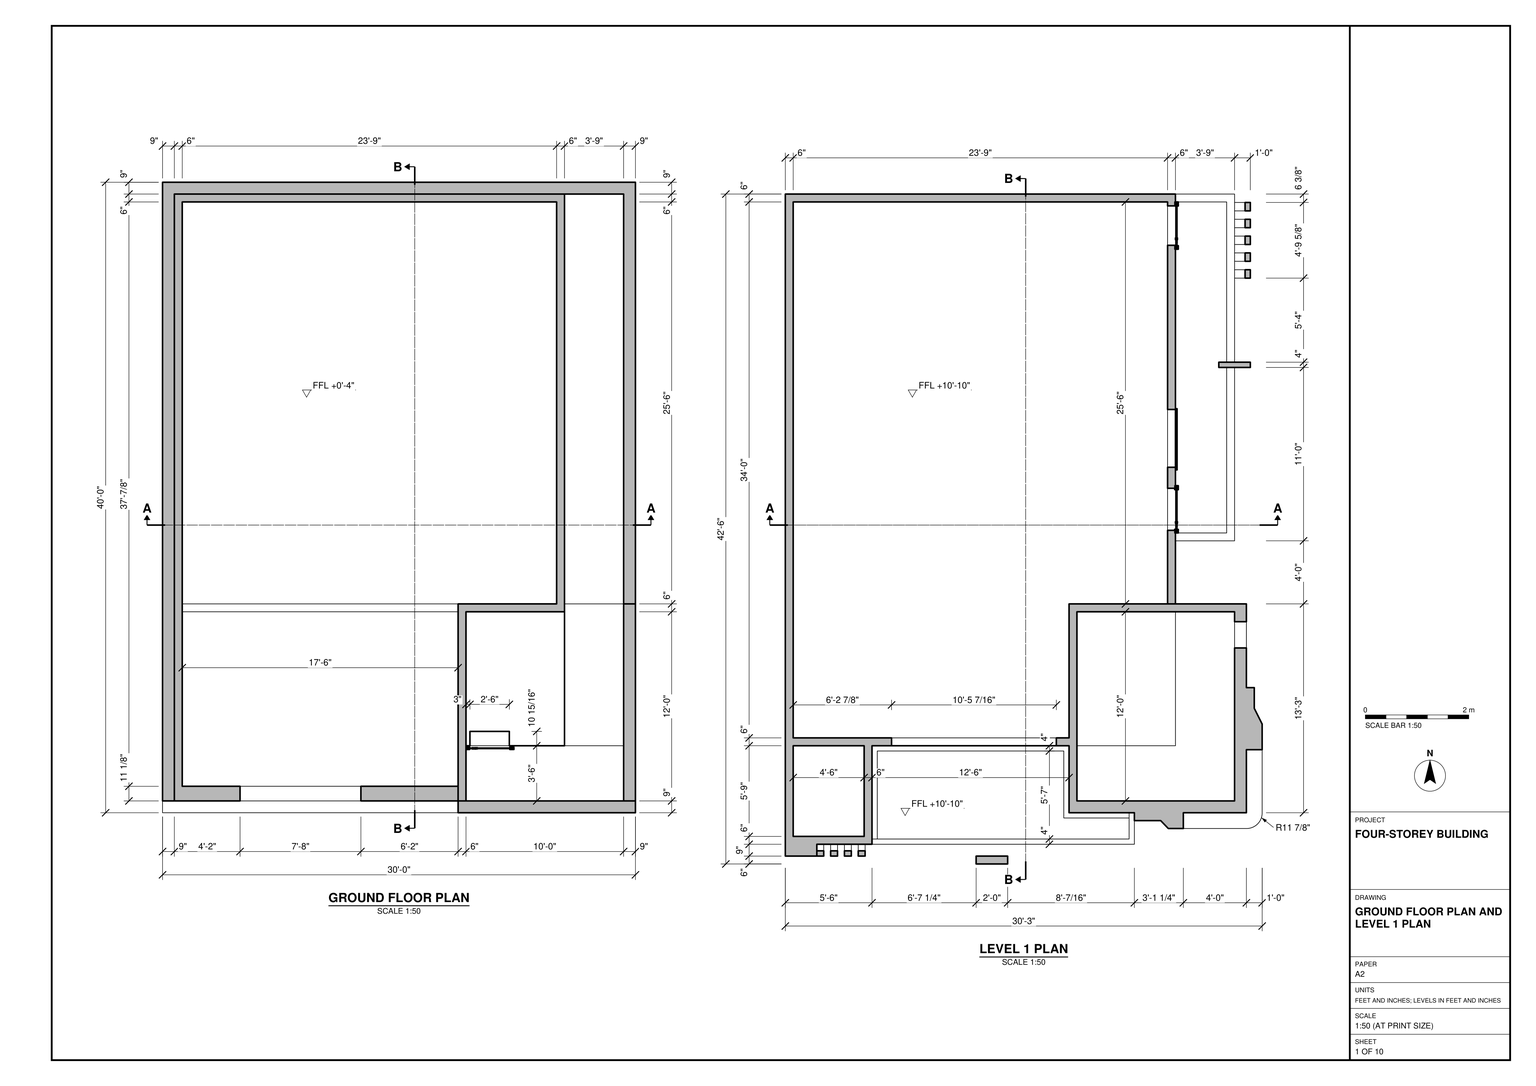
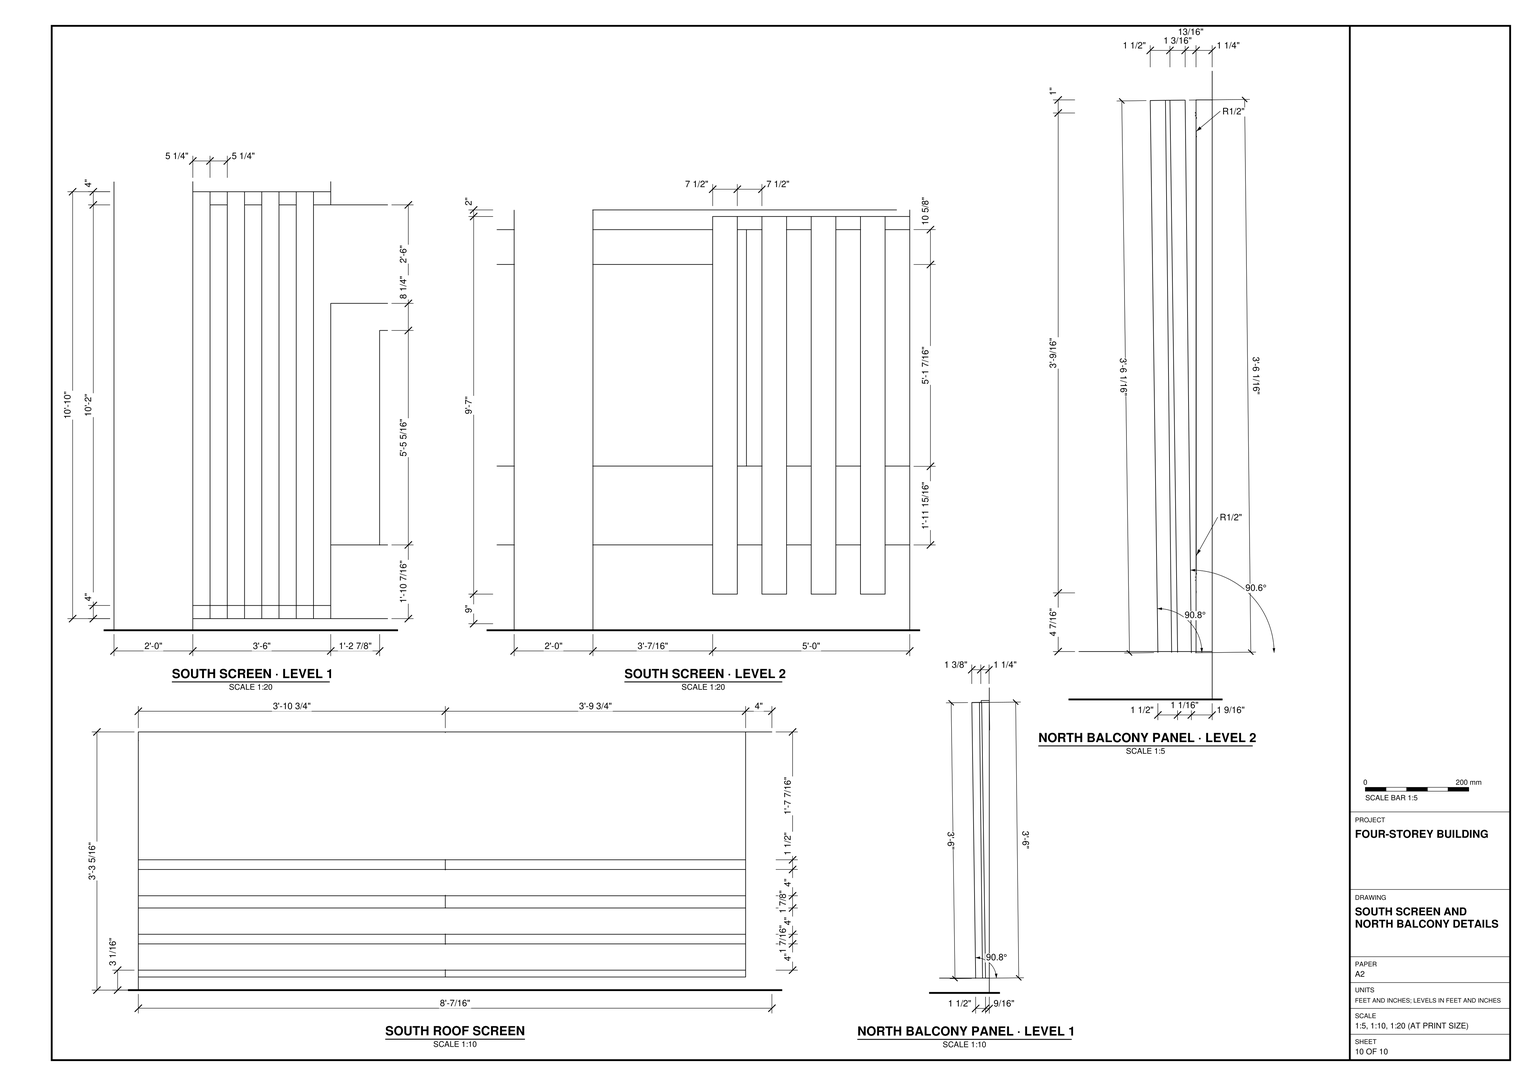
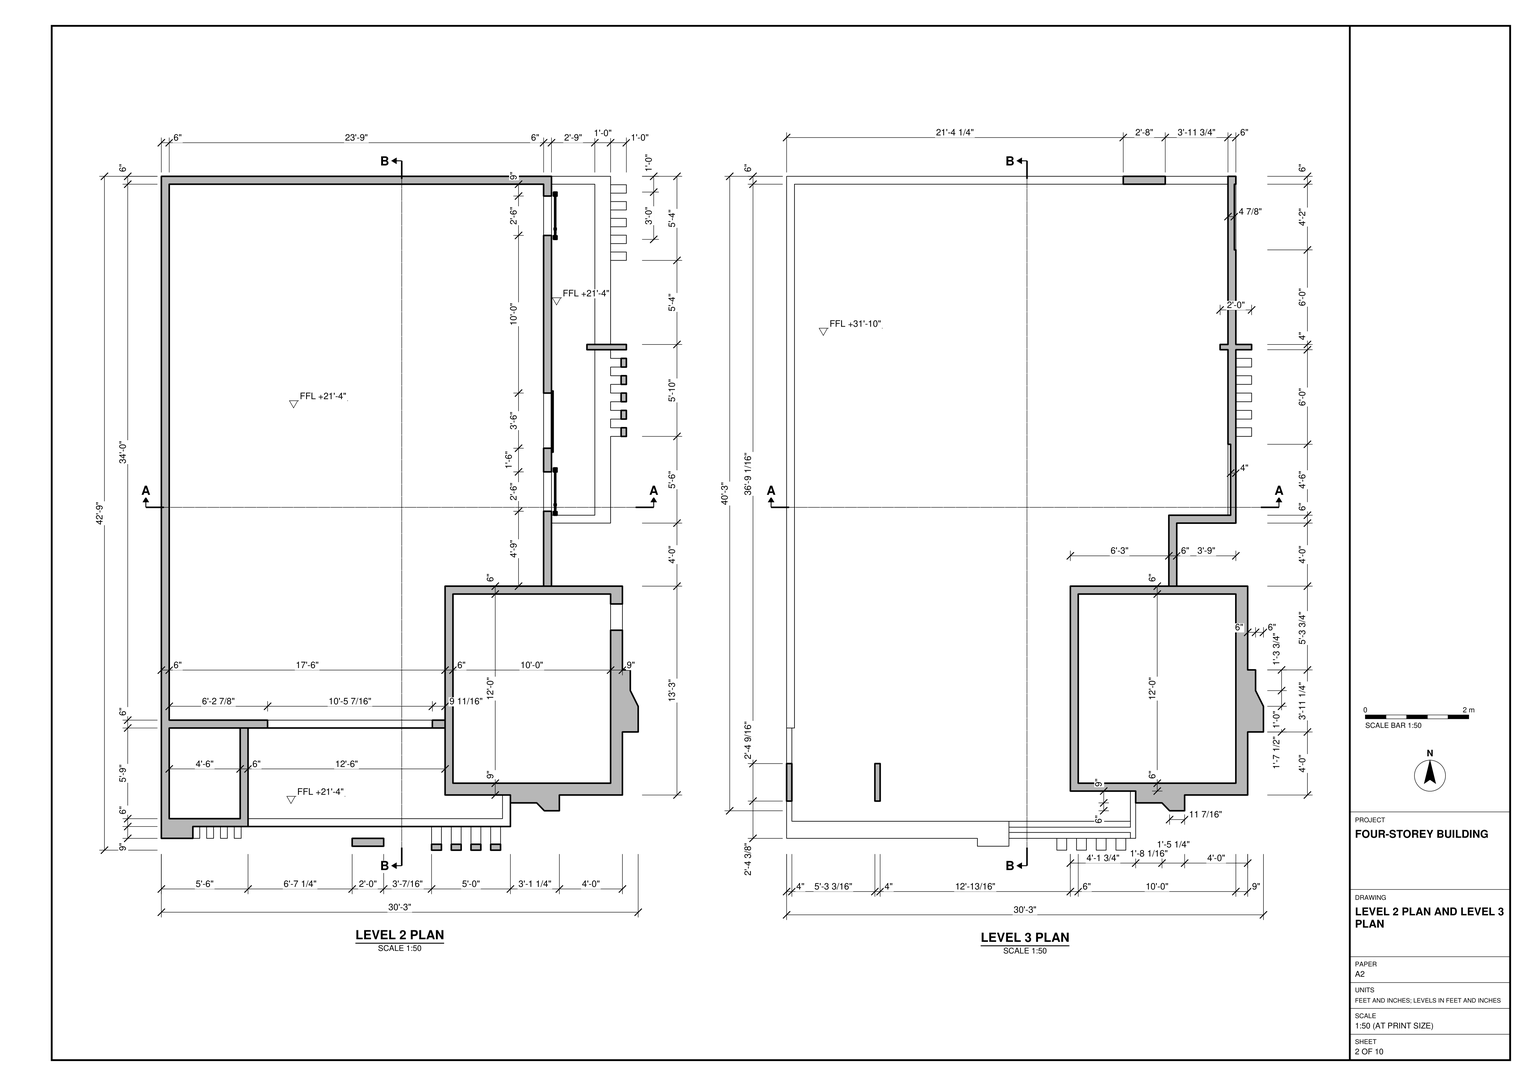
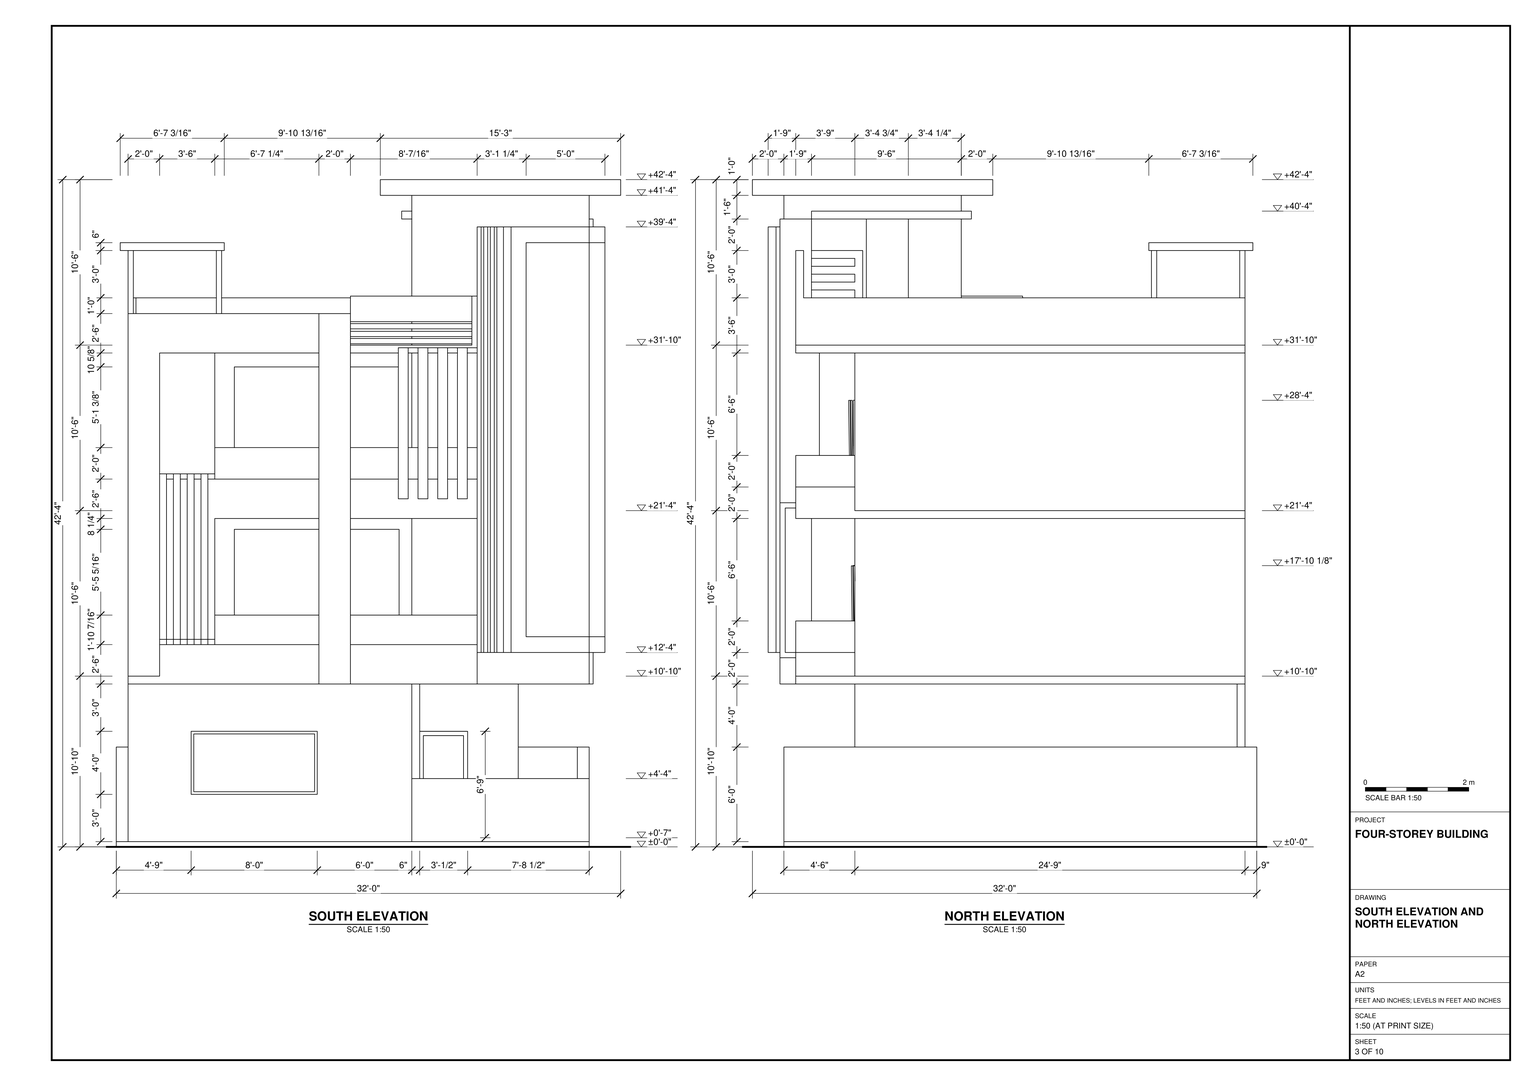
Use task_files/diagram_01.pdf to build the four-storey building in SketchUp. Work in feet and inches. The overall extents, including projections, are 32'-0" east to west, 43'-6" north to south and 42'-4" high. Set the ground datum at ±0'-0" and the upper levels at +10'-10", +21'-4" and +31'-10".

Build each floor from its own plan. Place the wide opening in the south ground-floor wall, align the southeast bay through the upper levels and follow the stepped outline at level 3. Use the wall thicknesses dimensioned on the plans, including 6" and 9" where shown. Place the doors and window units in their drawn openings. Use the plans and sections together for floor slabs, balconies, stairs where shown, and the roof. Match the south screens, south roof screen and north balcony panels to the details on sheet 10; the screen layout changes between levels 1 and 2.

Include built-in joinery and main furniture only where shown. Decor and loose items may be any suitable library components. Keep shell elements such as walls, slabs and roof, and each furniture or joinery piece, in separate groups or components. Use components for repeated parts. Save one SketchUp model as output_files/four_storey_building_with_balconies_and_facade_screens.skp.

# SketchUp Ruby script. Lengths in inches.
U = 1.inch
M = Sketchup.active_model
def pt(a) = Geom::Point3d.new(a.map { |v| v * U })
def face(e, loops, mat)
  f = e.add_face(loops[0].map { |a| pt(a) })
  loops[1..].each { |l| e.add_face(l.map { |a| pt(a) }).erase! }
  f.material = f.back_material = mat if mat
  f
end
# faces: each face lists its corners as indices into pts; further lists are holes
def faces(e, pts, list, mat = nil) = list.each { |f| face(e, (f[0].is_a?(Array) ? f : [f]).map { |l| l.map { |i| pts[i] } }, mat) }
# xy, xz, yz: faces in a plane at the given z, y or x. An outline is a flat list of corners, or four numbers for a rectangle; further outlines are holes
def ring(l) = l.size == 4 ? [[l[0], l[1]], [l[2], l[1]], [l[2], l[3]], [l[0], l[3]]] : l.each_slice(2).to_a
def flat(e, list, mat, &to3) = list.each { |f| face(e, (f[0].is_a?(Array) ? f : [f]).map { |l| ring(l).map { |u, v| to3.(u, v) } }, mat) }
def xy(e, z, list, mat = nil) = flat(e, list, mat) { |x, y| [x, y, z] }
def xz(e, y, list, mat = nil) = flat(e, list, mat) { |x, z| [x, y, z] }
def yz(e, x, list, mat = nil) = flat(e, list, mat) { |y, z| [x, y, z] }
def lines(e, pts, list) = list.each { |a, b| e.add_line(pt(pts[a]), pt(pts[b])) }
# prism: a flat outline (further loops are holes) pulled along v
def prism(e, loops, v, mat = nil)
  f = face(e, loops, mat); d = Geom::Vector3d.new(v.map { |x| x * U })
  f.pushpull(f.normal.samedirection?(d) ? d.length : -d.length)
end
def box(e, o, s, mat = nil) = prism(e, [[o, [o[0] + s[0], o[1], o[2]], [o[0] + s[0], o[1] + s[1], o[2]], [o[0], o[1] + s[1], o[2]]]], [0, 0, s[2]], mat)
def at(x, y, z, deg = 0) = Geom::Transformation.translation(pt([x, y, z])) * Geom::Transformation.rotation(ORIGIN, Z_AXIS, deg.degrees)
def axes(o, x, y, z) = Geom::Transformation.new([*x, 0, *y, 0, *z, 0, *pt(o).to_a, 1])
def part(name) = M.definitions.add(name)
# library, detail: a bought-in or finely detailed component or shape, given as its bounding box
def library(name, o, s) = part(name).tap { |d| box(d.entities, o, s) }
def detail(e, o, s) = box(e.add_group.entities, o, s)
def put(e, d, t, mat = nil) = e.add_instance(d, t).tap { |i| i.material = mat if mat }
def group(e, t, mat = nil) = e.add_group.tap { |g| g.transformation = t; g.material = mat if mat }.entities
root = M.entities
M.materials.add("C03_Honey_Glow").color = [255, 178, 101]
M.materials.add("C05_Golden_Blaze").color = [255, 123, 0]
M.materials.add("Carpet_04_1K").color = [43, 65, 85]
M.materials.add("D01_Frost_White").color = [255, 242, 206]
M.materials.add("Glass_Basic_01").color = [255, 228, 98]
M.materials["Glass_Basic_01"].alpha = 0.25
M.materials.add("M04_Stone_Frost").color = [142, 142, 142]
M.materials.add("Marble_01_1K").color = [230, 221, 211]
M.materials.add("Plywood_08_1K").color = [202, 166, 113]
M.materials.add("ThomThom - Waistcoat1").color = [242, 242, 242]
M.materials.add("ThomThom - Waistcoat2").color = [178, 178, 177]
M.materials.add("Wood_Veneer_15_1K").color = [103, 69, 45]
M.materials.add("mat_03").color = [63, 24, 24]
c1 = library("porta+4",[0.2,-5.42,1.33],[46.55,4.72,83.21])
c2 = library("mesh-164",[-1582.71,-3144.16,-23.22],[2366.42,2227.34,65.81])
c3 = part("Group13")
put(c3.entities,c2,at(294.66,859.51,3.5))
box(root,[201,21,492],[183,204,12],"M04_Stone_Frost")
xy(root,-4,[[0,42,360,522]])
xy(root,414,[[265.28,507,297.25,513]])
xy(root,474,[[217.28,357,339,507],[217.28,507,265.28,513],[265.28,507,297.25,513],[297.25,507,339,519],[217.28,513,297.25,519]])
xy(root,480,[[217.28,357,339,519]],"M04_Stone_Frost")
xz(root,42,[[0,-4,360,0]])
xz(root,357,[[217.28,474,339,480]],"M04_Stone_Frost")
xz(root,507,[[265.28,414,297.25,474]],"mat_03")
xz(root,513,[[265.28,414,297.25,474]],"mat_03")
xz(root,519,[[217.28,474,339,480]],"M04_Stone_Frost")
xz(root,522,[[0,-4,360,0]])
yz(root,0,[[42,-4,522,0]])
yz(root,217.28,[[357,474,519,480]],"M04_Stone_Frost")
yz(root,265.28,[[507,414,513,474]],"mat_03")
yz(root,297.25,[[507,414,513,474]],"mat_03")
yz(root,339,[[357,474,519,480]],"M04_Stone_Frost")
yz(root,360,[[42,-4,522,0]])
g1 = group(root,at(0,42,0),"D01_Frost_White")
box(g1,[15,-18,126],[54,69,120])
xy(g1,0,[[0,0,225,9],[9,9,225,9,225,20.15,15,20.15,15,465,300,465,300,159,225,159,225,51,231,51,231,153,306,153,306,471,9,471],[225,9,231,51],[231,9,351,51],[351,9,360,159],
  [15,20.15,225,153],[231,51,306,153],[306,51,351,159],[15,153,225,159],[15,159,300,465],
  [306,159,351,471]])
xy(g1,3,[[234,51,264,61.91]])
xy(g1,38,[[59,9,151,20.15]])
xy(g1,48,[[225,0,360,9]])
xy(g1,48,[[351,9,360,159]],"Plywood_08_1K")
xy(g1,72,[[0,9,9,9,9,471,351,471,351,159,360,159,360,480,0,480]])
xy(g1,81,[[234,51,264,61.91]])
xy(g1,82,[[59,9,151,20.15]])
xy(g1,120,[[9,-24,9,9,351,9,351,153,306,153,306,159,360,159,360,0,274.72,0,274.72,-24],[9,9,225,9,225,20.15,15,20.15,15,57,9,57],[225,9,231,51],[231,9,231,51,306,51,306,153,351,153,351,9],[15,20.15,15,465,300,465,300,159,225,159,225,20.15],
  [9,57,15,159],[9,159,15,471],[300,159,306,465],[306,207,306,465,351,465,351,343,363,343,363,339,351,339,351,207],[15,465,306,471],
  [306,465,351,471]])
xy(g1,120,[[154.26,-39,178.26,-33]],"M04_Stone_Frost")
xy(g1,126,[[9,-33,33,-24],[75,-20,79,-20,79,47,221,47,221,-4,270.72,-4,270.72,0,225,0,225,51,75,51],[79,-20,270.72,-20,270.72,-4,221,-4,221,47,79,47],[15,57,225,57,225,159,300,159,300,465,15,465],[306,213,345,213,345,339,339,339,339,343,345,343,345,465,306,465]])
xy(g1,128,[[300,215,306,247]])
xy(g1,129,[[300,432,306,462]])
xy(g1,136.09,[[89.88,51,215.3125,57]])
xy(g1,140,[[351,407,363,413.4],[351,419.8,363,426.2],[351,432.6,363,439],[351,445.4,363,451.8],[351,458.2,363,464.6]],"Marble_01_1K")
xy(g1,144,[[300.55,-12,300.55,-6,274.72,-6,274.72,0,360,0,360,95.25,366,95.25,366,79.5,372,67.5,372,-0.38,371.98,-0.76,371.96,-1.13,371.92,-1.51,371.87,-1.88,371.81,-2.26,371.65,-3,371.55,-3.36,371.44,-3.72,371.32,-4.08,371.19,-4.4375,371.05,-4.79,370.9,-5.13,370.73,-5.47,370.55,-5.81,370.37,-6.14,369.97,-6.78,369.75,-7.09,369.52,-7.39,369.29,-7.68,369.04,-7.97,368.79,-8.25,368.25,-8.79,367.97,-9.04,367.68,-9.29,367.39,-9.52,367.09,-9.75,366.78,-9.97,366.14,-10.37,365.81,-10.55,365.47,-10.73,365.13,-10.9,364.79,-11.05,364.4375,-11.19,364.08,-11.32,363.72,-11.44,363.36,-11.55,363,-11.65,362.26,-11.81,361.88,-11.87,361.51,-11.92,361.13,-11.96,360.76,-11.98,360.38,-12],[300.55,-12,294.76,-6,300.55,-6],[306,207,351,207,351,339,345,339,345,213,306,213],[345,343,351,343,351,471,306,471,306,465,345,465],[351,407,359,413.4],
  [351,419.8,359,426.2],[351,432.6,359,439],[351,445.4,359,451.8],[351,458.2,359,464.6]])
xy(g1,150,[[33,-33,38.25,-24],[43.5,-33,48.75,-24],[54,-33,59.25,-24],[64.5,-33,69.75,-24],[75,-24,274.72,-24,274.72,0,270.72,0,270.72,-20,75,-20]])
xy(g1,154,[[33,-29,38.25,-24],[43.5,-29,48.75,-24],[54,-29,59.25,-24],[64.5,-29,69.75,-24]])
xy(g1,156,[[312,-12,360.38,-12,360.76,-11.98,361.13,-11.96,361.51,-11.92,361.88,-11.87,362.26,-11.81,363,-11.65,363.36,-11.55,363.72,-11.44,364.08,-11.32,364.4375,-11.19,364.79,-11.05,365.13,-10.9,365.47,-10.73,365.81,-10.55,366.14,-10.37,366.78,-9.97,367.09,-9.75,367.39,-9.52,367.68,-9.29,367.97,-9.04,368.25,-8.79,368.79,-8.25,369.04,-7.97,369.29,-7.68,369.52,-7.39,369.75,-7.09,369.97,-6.78,370.37,-6.14,370.55,-5.81,370.73,-5.47,370.9,-5.13,371.05,-4.79,371.19,-4.4375,371.32,-4.08,371.44,-3.72,371.55,-3.36,371.65,-3,371.81,-2.26,371.87,-1.88,371.92,-1.51,371.96,-1.13,371.98,-0.76,372,-0.38,372,48,360,48,360,0,312,0]],"M04_Stone_Frost")
xy(g1,158,[[351,125.45,360,145.45]])
xy(g1,164,[[300,263,306,307]])
xy(g1,202,[[351,125.45,360,145.45]])
xy(g1,207,[[300,432,306,462]])
xy(g1,208,[[300,215,306,247],[300,263,306,307]])
xy(g1,237.75,[[89.88,51,215.3125,57]])
xy(g1,246,[[9,57,15,159],[15,57,15,465,300,465,300,159,225,159,225,57],[9,159,15,471],[300,159,306,465],[15,465,306,471],
  [306,465,351,471]])
xy(g1,246,[[75,-24,75,51,225,51,225,0,274.72,0,274.72,-24]],"C05_Golden_Blaze")
xy(g1,246,[[306,207,306,465,351,465,351,343,339,343,339,339,351,339,351,207]],"Wood_Veneer_15_1K")
xy(g1,252,[[15,-18,69,51],[75,-18,268.72,-18,268.72,0,225,0,225,51,75,51],[15,57,225,57,225,159,300,159,300,465,15,465],[306,213,339,213,339,339,333,339,333,343,339,343,339,465,306,465]])
xy(g1,254,[[351,407,359,413.4],[351,419.8,359,426.2],[351,432.6,359,439],[351,445.4,359,451.8],[351,458.2,359,464.6]])
xy(g1,255,[[300,216,306,246],[300,426,306,456]])
xy(g1,258,[[351,407,363,413.4],[351,419.8,363,426.2],[351,432.6,363,439],[351,445.4,363,451.8],[351,458.2,363,464.6]])
xy(g1,259.73,[[89.88,51,215.3125,57]])
xy(g1,261,[[214.71,-42,222.21,-24],[229.72,-42,237.22,-24],[244.72,-42,252.22,-24],[259.72,-42,267.22,-24]])
xy(g1,265,[[214.71,-37.5,222.21,-24],[229.72,-37.5,237.22,-24],[244.72,-37.5,252.22,-24],[259.72,-37.5,267.22,-24]])
xy(g1,266,[[351,273,363,279.6],[351,286.2,363,292.8],[351,299.4,363,306],[351,312.6,363,319.2],[351,325.8,363,332.4]])
xy(g1,270,[[339,343,351,343,351,471,306,471,306,465,339,465]])
xy(g1,270,[[306,207,351,207,351,273,359,273,359,279.6,351,279.6,351,286.2,359,286.2,359,292.8,351,292.8,351,299.4,359,299.4,359,306,351,306,351,312.6,359,312.6,359,319.2,351,319.2,351,325.8,359,325.8,359,332.4,351,332.4,351,339,339,339,339,213,306,213]],"D01_Frost_White")
xy(g1,276,[[33,-29,38.25,-24],[43.5,-29,48.75,-24],[54,-29,59.25,-24],[64.5,-29,69.75,-24],[75,-24,274.72,-24,274.72,0,268.72,0,268.72,-18,75,-18]])
xy(g1,280,[[33,-33,38.25,-24],[43.5,-33,48.75,-24],[54,-33,59.25,-24],[64.5,-33,69.75,-24]])
xy(g1,290,[[351,125.45,360,145.45]])
xy(g1,291,[[300,264,306,306]])
xy(g1,333,[[300,216,306,246],[300,264,306,306],[300,426,306,456]])
xy(g1,334,[[351,125.45,360,145.45]])
xy(g1,361.39,[[89.88,51,215.3125,57]])
xy(g1,372,[[15,-18,69,51],[9,57,15,159],[15,57,15,465,300,465,300,159,225,159,225,57],[9,159,15,471],[300,159,306,465],
  [306,207,351,213],[15,465,306,471],[306,465,351,471]])
xy(g1,372,[[214.71,-37.5,214.71,-33,33,-33,33,-24,75,-24,75,51,225,51,225,0,274.72,0,274.72,-33,267.22,-33,267.22,-37.5,259.72,-37.5,259.72,-33,252.22,-33,252.22,-37.5,244.72,-37.5,244.72,-33,237.22,-33,237.22,-37.5,229.72,-37.5,229.72,-33,222.21,-33,222.21,-37.5]],"C05_Golden_Blaze")
xy(g1,372,[[306,213,306,465,351,465,351,343,333,343,333,339,351,339,351,213]],"Wood_Veneer_15_1K")
xy(g1,376,[[214.71,-42,222.21,-33],[229.72,-42,237.22,-33],[244.72,-42,252.22,-33],[259.72,-42,267.22,-33]])
xy(g1,378,[[178.26,-33,270.72,-20],[[13,-20,270.72,-20,270.72,3,225,3,225,159,300,159,300,213,345,213,345,339,339,339,339,343,345,343,345,465,15,465,15,51,13,51],[76.21,-4.625,80.21,23.93]]])
xy(g1,379.04,[[178.26,-28.51,270.72,-24.51]])
xy(g1,380,[[351,273,359,279.6],[351,286.2,359,292.8],[351,299.4,359,306],[351,312.6,359,319.2],[351,325.8,359,332.4]])
xy(g1,383.04,[[178.26,-28.51,270.72,-24.51]],"C03_Honey_Glow")
xy(g1,384,[[351,273,363,279.6],[351,286.2,363,292.8],[351,299.4,363,306],[351,312.6,363,319.2],[351,325.8,363,332.4]],"Marble_01_1K")
xy(g1,384.51,[[178.26,-28.51,270.72,-24.51]])
xy(g1,388.51,[[178.26,-28.51,270.72,-24.51]],"C03_Honey_Glow")
xy(g1,390.37,[[178.26,-28.51,270.72,-24.51]])
xy(g1,394.37,[[178.26,-28.51,270.72,-24.51]],"C03_Honey_Glow")
xy(g1,395.85,[[178.26,-28.51,270.72,-24.51]])
xy(g1,402,[[154.26,-39,178.26,-39,178.26,-20,13,-20,13,-4.625,9,-4.625,9,-33,154.26,-33],[9,23.93,13,51]])
xy(g1,414,[[9,51,15,51,15,465,345,465,345,471,9,471],[300,159,306,207],[306,207,351,207,351,267,345,267,345,213,306,213],[345,415,351,465]])
xy(g1,415.3125,[[270.72,-33,274.72,-33,274.72,3,270.72,3,270.72,-24.51,178.26,-24.51,178.26,-28.51,270.72,-28.51]],"C03_Honey_Glow")
xy(g1,419.87,[[300,159,306,207]])
xy(g1,420,[[306,207,306,213,347,213,347,267,351,267,351,207],[345,415,349.86,465]])
xy(g1,426,[[300,159,306,207],[306,207,351,207,351,267,347,267,347,213,306,213],[345,415,349.86,465]],"C03_Honey_Glow")
xy(g1,432,[[300,159,306,207],[306,207,306,213,347,213,347,267,351,267,351,207],[345,415,349.86,465]])
xy(g1,438,[[300,159,306,207],[306,207,351,207,351,267,347,267,347,213,306,213],[345,415,349.86,465]],"C03_Honey_Glow")
xy(g1,444,[[300,159,306,207],[306,207,306,213,347,213,347,267,351,267,351,207],[345,415,349.86,465]])
xy(g1,450,[[9,-4.625,13,23.93],[76.21,-4.625,80.21,23.93],[80.21,-4.625,82.21,23.93],[345,267,351,339],[345,343,351,343,351,415,349.86,415,349.86,465,345,465],
  [345,465,351,471]])
xy(g1,450,[[300,159,306,159,306,207,351,207,351,267,347,267,347,213,300,213]],"C03_Honey_Glow")
xy(g1,450,[[3,-4.625,9,23.93],[13,-4.625,76.21,23.93]],"M04_Stone_Frost")
xy(g1,456,[[312,-12,312,0,360,0,360,48,372,48,372,0,371.98,-0.37,371.9,-1.11,371.78,-1.85,371.7,-2.21,371.61,-2.57,371.51,-2.93,371.4,-3.29,371.28,-3.64,371.15,-3.99,371.01,-4.33,370.86,-4.68,370.7,-5.01,370.53,-5.34,370.35,-5.67,370.16,-5.99,369.76,-6.61,369.54,-6.91,369.3125,-7.21,369.08,-7.5,368.58,-8.06,368.06,-8.58,367.5,-9.08,367.21,-9.3125,366.91,-9.54,366.61,-9.76,365.99,-10.16,365.67,-10.35,365.34,-10.53,365.01,-10.7,364.68,-10.86,364.33,-11.01,363.99,-11.15,363.64,-11.28,363.29,-11.4,362.93,-11.51,362.57,-11.61,362.21,-11.7,361.85,-11.78,361.11,-11.9,360.37,-11.98,360,-12]])
xy(g1,456,[[3,-4.625,82.21,23.93]],"M04_Stone_Frost")
xy(g1,468,[[300.55,-12,360,-12,360.37,-11.98,361.11,-11.9,361.85,-11.78,362.21,-11.7,362.57,-11.61,362.93,-11.51,363.29,-11.4,363.64,-11.28,363.99,-11.15,364.33,-11.01,364.68,-10.86,365.01,-10.7,365.34,-10.53,365.67,-10.35,365.99,-10.16,366.61,-9.76,366.91,-9.54,367.21,-9.3125,367.5,-9.08,368.06,-8.58,368.58,-8.06,369.08,-7.5,369.3125,-7.21,369.54,-6.91,369.76,-6.61,370.16,-5.99,370.35,-5.67,370.53,-5.34,370.7,-5.01,370.86,-4.68,371.01,-4.33,371.15,-3.99,371.28,-3.64,371.4,-3.29,371.51,-2.93,371.61,-2.57,371.7,-2.21,371.78,-1.85,371.9,-1.11,371.98,-0.37,372,0,372,67.5,366,79.5,366,95.25,360,95.25,360,3,274.72,3,274.72,-6,294.76,-6]],"M04_Stone_Frost")
xy(g1,474,[[339,339,363,343]],"Wood_Veneer_15_1K")
xy(g1,492,[[[225,3,360,159],[231,9,351,153]]])
xz(g1,-42,[[214.71,261,222.21,376],[229.72,261,237.22,376],[244.72,261,252.22,376],[259.72,261,267.22,376]],"Marble_01_1K")
xz(g1,-39,[[154.26,120,178.26,402]],"M04_Stone_Frost")
xz(g1,-37.5,[[214.71,265,222.21,372],[229.72,265,237.22,372],[244.72,265,252.22,372],[259.72,265,267.22,372]])
xz(g1,-33,[[33,150,38.25,154],[43.5,150,48.75,154],[54,150,59.25,154],[64.5,150,69.75,154],[222.21,372,229.72,376],
  [237.22,372,244.72,376],[252.22,372,259.72,376],[267.22,372,274.72,376]])
xz(g1,-33,[[9,126,33,126,33,372,154.26,372,154.26,402,9,402],[178.26,372,214.71,372,214.71,376,274.72,376,274.72,415.3125,270.72,415.3125,270.72,378,178.26,378]],"Carpet_04_1K")
xz(g1,-33,[[154.26,120,178.26,372]],"M04_Stone_Frost")
xz(g1,-33,[[33,154,38.25,280],[43.5,154,48.75,280],[54,154,59.25,280],[64.5,154,69.75,280]],"Marble_01_1K")
xz(g1,-29,[[33,154,38.25,276],[43.5,154,48.75,276],[54,154,59.25,276],[64.5,154,69.75,276]])
xz(g1,-28.51,[[178.26,379.04,270.72,383.04],[178.26,384.51,270.72,388.51],[178.26,390.37,270.72,394.37],[178.26,395.85,270.72,415.3125]],"C03_Honey_Glow")
xz(g1,-24.51,[[178.26,379.04,270.72,383.04],[178.26,384.51,270.72,388.51],[178.26,390.37,270.72,394.37],[178.26,395.85,270.72,415.3125]],"C03_Honey_Glow")
xz(g1,-24,[[38.25,150,43.5,154],[48.75,150,54,154],[59.25,150,64.5,154],[69.75,150,75,154],[38.25,276,43.5,280],
  [48.75,276,54,280],[59.25,276,64.5,280],[69.75,276,75,280]])
xz(g1,-24,[[9,120,274.72,120,274.72,150,33,150,33,126,9,126],[[33,154,75,154,75,246,274.72,246,274.72,276,33,276],[214.71,261,222.21,265],[229.72,261,237.22,265],[244.72,261,252.22,265],[259.72,261,267.22,265]],[33,280,75,372]],"D01_Frost_White")
xz(g1,-24,[[75,150,274.72,172.45],[75,276,274.72,300]],"Glass_Basic_01")
xz(g1,-20,[[75,126,79,150],[79,126,270.72,150],[13,378,178.26,402]])
xz(g1,-18,[[15,252,69,372],[75,252,268.72,276]])
xz(g1,-12,[[300.55,144,360,144,360,156,312,156,312,456,360,456,360,468,300.55,468],[360,144,360.38,156]],"M04_Stone_Frost")
xz(g1,-6,[[277.73,144,279.73,468],[282.74,144,284.74,468],[287.75,144,289.75,468]])
xz(g1,-6,[[274.72,144,277.73,468],[279.73,144,282.74,468],[284.74,144,287.75,468],[289.75,144,294.76,468]],"M04_Stone_Frost")
xz(g1,-4.625,[[76.21,378,80.21,450],[9,402,13,450],[3,450,82.21,456]],"M04_Stone_Frost")
xz(g1,0,[[225,246,274.72,246,274.72,276,268.72,276,268.72,252,225,252]])
xz(g1,0,[[225,126,270.72,126,270.72,150,274.72,150,274.72,246,225,246],[225,252,268.72,252,268.72,276,274.72,276,274.72,372,225,372]],"D01_Frost_White")
xz(g1,0,[[312,156,360,456]],"Glass_Basic_01")
xz(g1,0,[[274.72,120,360,144]],"M04_Stone_Frost")
xz(g1,0,[[225,0,360,48]],"ThomThom - Waistcoat1")
xz(g1,3,[[225,378,270.72,378,270.72,415.3125,274.72,415.3125,274.72,468,360,468,360,492,225,492]],"M04_Stone_Frost")
xz(g1,9,[[0,0,9,72],[225,0,231,48],[231,0,351,48],[[57,36,153,84],[59,38,151,82]],[225,48,231,120],
  [231,120,351,492]])
xz(g1,9,[[351,0,360,48]],"Plywood_08_1K")
xz(g1,9,[[[9,0,225,120],[57,36,153,84]]],"ThomThom - Waistcoat1")
xz(g1,20.15,[[[15,0,225,120],[59,38,151,82]]])
xz(g1,23.93,[[76.21,378,80.21,450],[9,402,13,450]])
xz(g1,23.93,[[3,450,82.21,456]],"M04_Stone_Frost")
xz(g1,48,[[360,156,372,456]],"M04_Stone_Frost")
xz(g1,51,[[[231,0,267,84],[234,3,264,81]],[15,252,69,372],[69,252,75,372],[13,378,15,378,15,414,9,414,9,402,13,402]])
xz(g1,51,[[[75,126,225,246],[89.88,136.09,215.3125,237.75]],[[75,252,225,372],[89.88,259.73,215.3125,361.39]]],"D01_Frost_White")
xz(g1,51,[[89.88,136.09,215.3125,237.75],[89.88,259.73,215.3125,361.39]],"Glass_Basic_01")
xz(g1,51,[[267,0,306,0,306,120,231,120,231,84,267,84]],"ThomThom - Waistcoat1")
xz(g1,57,[[[15,126,225,246],[89.88,136.09,215.3125,237.75]],[[15,252,225,372],[89.88,259.73,215.3125,361.39]]])
xz(g1,61.91,[[234,3,264,81]])
xz(g1,95.25,[[360,144,366,468]])
xz(g1,125.45,[[351,158,360,202],[351,290,360,334]])
xz(g1,145.45,[[351,158,360,202],[351,290,360,334]])
xz(g1,153,[[231,0,306,0,306,120,351,120,351,492,231,492]])
xz(g1,159,[[225,0,300,120],[351,48,360,72],[225,120,225,126,300,126,300,246,306,246,306,120],[225,126,300,246],[225,246,225,252,300,252,300,372,306,372,306,246],
  [225,252,300,372],[225,372,225,378,300,378,300,414,306,414,306,372],[300,414,306,419.87],[300,419.87,306,426],[300,426,306,432],
  [300,432,306,438],[300,438,306,444],[300,444,306,450]])
xz(g1,159,[[306,120,306,450,300,450,300,378,225,378,225,492,360,492,360,120]],"M04_Stone_Frost")
xz(g1,159,[[351,0,360,48]],"Plywood_08_1K")
xz(g1,207,[[300,414,306,419.87],[300,426,306,432],[300,438,306,444]])
xz(g1,207,[[306,420,351,426],[306,432,351,438],[306,444,351,450]],"C03_Honey_Glow")
xz(g1,207,[[306,120,351,144],[306,246,351,270],[306,372,351,414]],"D01_Frost_White")
xz(g1,207,[[306,144,351,168],[306,270,351,294]],"Glass_Basic_01")
xz(g1,213,[[306,126,345,144],[306,252,339,270],[300,378,300,450,347,450,347,444,306,444,306,438,347,438,347,432,306,432,306,426,347,426,347,420,306,420,306,414,345,414,345,378]])
xz(g1,215,[[300,128,306,144],[300,144,306,208]])
xz(g1,216,[[300,255,306,270],[300,270,306,333]])
xz(g1,246,[[300,255,306,333]])
xz(g1,247,[[300,128,306,208]])
xz(g1,263,[[300,164,306,208]])
xz(g1,264,[[300,291,306,333]])
xz(g1,267,[[345,414,351,414,351,420,347,420,347,426,351,426,351,432,347,432,347,438,351,438,351,444,347,444,347,450,345,450]])
xz(g1,273,[[351,266,363,266,363,384,351,384,351,380,359,380,359,270,351,270]],"Marble_01_1K")
xz(g1,279.6,[[351,266,351,270,359,270,359,380,351,380,351,384,363,384,363,266]],"Marble_01_1K")
xz(g1,286.2,[[351,266,363,266,363,384,351,384,351,380,359,380,359,270,351,270]],"Marble_01_1K")
xz(g1,292.8,[[351,266,351,270,359,270,359,380,351,380,351,384,363,384,363,266]],"Marble_01_1K")
xz(g1,299.4,[[351,266,363,266,363,384,351,384,351,380,359,380,359,270,351,270]],"Marble_01_1K")
xz(g1,306,[[300,291,306,333]])
xz(g1,306,[[351,266,351,270,359,270,359,380,351,380,351,384,363,384,363,266]],"Marble_01_1K")
xz(g1,307,[[300,164,306,208]])
xz(g1,312.6,[[351,266,363,266,363,384,351,384,351,380,359,380,359,270,351,270]],"Marble_01_1K")
xz(g1,319.2,[[351,266,351,270,359,270,359,380,351,380,351,384,363,384,363,266]],"Marble_01_1K")
xz(g1,325.8,[[351,266,363,266,363,384,351,384,351,380,359,380,359,270,351,270]],"Marble_01_1K")
xz(g1,332.4,[[351,266,351,270,359,270,359,380,351,380,351,384,363,384,363,266]],"Marble_01_1K")
xz(g1,339,[[351,120,363,120,363,474,339,474,339,378,345,378,345,450,351,450,351,372,333,372,333,252,339,252,339,270,351,270,351,246,339,246,339,126,345,126,345,144,351,144]],"Wood_Veneer_15_1K")
xz(g1,343,[[351,120,351,144,345,144,345,126,339,126,339,246,351,246,351,270,339,270,339,252,333,252,333,372,351,372,351,450,345,450,345,378,339,378,339,474,363,474,363,120]],"Wood_Veneer_15_1K")
xz(g1,407,[[351,140,363,140,363,258,351,258,351,254,359,254,359,144,351,144]],"Marble_01_1K")
xz(g1,413.4,[[351,140,351,144,359,144,359,254,351,254,351,258,363,258,363,140]],"Marble_01_1K")
xz(g1,415,[[345,414,349.86,420],[349.86,414,351,420],[349.86,420,351,426],[345,426,349.86,432],[349.86,426,351,432],
  [349.86,432,351,438],[345,438,349.86,444],[349.86,438,351,444],[349.86,444,351,450]])
xz(g1,419.8,[[351,140,363,140,363,258,351,258,351,254,359,254,359,144,351,144]],"Marble_01_1K")
xz(g1,426,[[300,255,306,333]])
xz(g1,426.2,[[351,140,351,144,359,144,359,254,351,254,351,258,363,258,363,140]],"Marble_01_1K")
xz(g1,432,[[300,129,306,207]])
xz(g1,432.6,[[351,140,363,140,363,258,351,258,351,254,359,254,359,144,351,144]],"Marble_01_1K")
xz(g1,439,[[351,140,351,144,359,144,359,254,351,254,351,258,363,258,363,140]],"Marble_01_1K")
xz(g1,445.4,[[351,140,363,140,363,258,351,258,351,254,359,254,359,144,351,144]],"Marble_01_1K")
xz(g1,451.8,[[351,140,351,144,359,144,359,254,351,254,351,258,363,258,363,140]],"Marble_01_1K")
xz(g1,456,[[300,255,306,333]])
xz(g1,458.2,[[351,140,363,140,363,258,351,258,351,254,359,254,359,144,351,144]],"Marble_01_1K")
xz(g1,462,[[300,129,306,144],[300,144,306,207]])
xz(g1,464.6,[[351,140,351,144,359,144,359,254,351,254,351,258,363,258,363,140]],"Marble_01_1K")
xz(g1,465,[[15,0,300,120],[15,126,300,246],[306,126,345,144],[15,252,300,372],[306,252,339,270],
  [15,378,345,414],[345,414,351,414,351,450,349.86,450,349.86,444,345,444,345,438,349.86,438,349.86,432,345,432,345,426,349.86,426,349.86,420,345,420]])
xz(g1,471,[[9,0,15,72],[15,0,306,72],[306,0,351,72],[9,72,15,120],[15,72,306,120],
  [9,126,306,246],[9,252,306,372],[9,378,9,414,345,414,345,450,351,450,351,378]])
xz(g1,471,[[9,120,351,126],[306,126,351,144],[9,246,9,252,306,252,306,270,351,270,351,246],[9,372,351,378]],"D01_Frost_White")
xz(g1,471,[[306,144,351,168],[306,270,351,294]],"Glass_Basic_01")
xz(g1,480,[[0,0,360,72]])
yz(g1,0,[[9,0,480,72]])
yz(g1,3,[[-4.625,450,23.93,456]],"M04_Stone_Frost")
yz(g1,9,[[9,0,471,72],[9,72,471,120],[-24,120,471,126],[-33,126,471,246],[-33,246,471,252],
  [-33,252,471,372],[-33,372,-33,402,-4.625,402,-4.625,450,23.93,450,23.93,402,51,402,51,378,471,378,471,372],[51,378,471,414]])
yz(g1,13,[[-20,378,47,402],[47,378,51,402],[-4.625,402,23.93,450]])
yz(g1,15,[[20.15,0,465,120],[57,126,465,246],[-18,252,51,372],[57,252,465,372],[51,378,57,414],
  [57,378,465,414]])
yz(g1,33,[[-33,126,-24,150],[-33,154,-29,246],[-29,154,-24,246],[-33,246,-29,252],[-29,246,-24,252],
  [-33,252,-29,276],[-29,252,-24,276]])
yz(g1,33,[[-33,280,-24,372]],"M04_Stone_Frost")
yz(g1,38.25,[[-33,150,-24,154],[-33,154,-29,154,-29,276,-24,276,-24,280,-33,280]])
yz(g1,43.5,[[-33,150,-24,154],[-33,154,-33,280,-24,280,-24,276,-29,276,-29,154]])
yz(g1,48.75,[[-33,150,-24,154],[-33,154,-29,154,-29,276,-24,276,-24,280,-33,280]])
yz(g1,54,[[-33,150,-24,154],[-33,154,-33,280,-24,280,-24,276,-29,276,-29,154]])
yz(g1,59,[[9,38,20.15,82]])
yz(g1,59.25,[[-33,150,-24,154],[-33,154,-29,154,-29,276,-24,276,-24,280,-33,280]])
yz(g1,64.5,[[-33,150,-24,154],[-33,154,-33,280,-24,280,-24,276,-29,276,-29,154]])
yz(g1,69,[[-18,252,51,372]])
yz(g1,69.75,[[-33,150,-24,154],[-33,154,-29,154,-29,276,-24,276,-24,280,-33,280]])
yz(g1,75,[[-20,126,51,126,51,246,-24,246,-24,150,-20,150],[-18,252,51,252,51,372,-24,372,-24,276,-18,276]],"C05_Golden_Blaze")
yz(g1,76.21,[[-4.625,378,23.93,450]],"M04_Stone_Frost")
yz(g1,80.21,[[-4.625,378,23.93,450]],"M04_Stone_Frost")
yz(g1,82.21,[[-4.625,450,23.93,456]],"M04_Stone_Frost")
yz(g1,89.88,[[51,136.09,57,237.75],[51,259.73,57,361.39]])
yz(g1,151,[[9,38,20.15,82]])
yz(g1,154.26,[[-39,120,-33,378],[-39,378,-33,402]],"M04_Stone_Frost")
yz(g1,178.26,[[-28.51,402,-24.51,415.3125]],"C03_Honey_Glow")
yz(g1,178.26,[[-39,120,-33,378],[[-39,378,-20,378,-20,402,-24.51,402,-24.51,395.85,-28.51,395.85,-28.51,402,-39,402],[-28.51,390.37,-24.51,394.37],[-28.51,384.51,-24.51,388.51],[-28.51,379.04,-24.51,383.04]]],"M04_Stone_Frost")
yz(g1,214.71,[[-42,261,-42,376,-33,376,-33,372,-37.5,372,-37.5,265,-24,265,-24,261]])
yz(g1,215.3125,[[51,136.09,57,237.75],[51,259.73,57,361.39]])
yz(g1,222.21,[[-42,261,-24,261,-24,265,-37.5,265,-37.5,372,-33,372,-33,376,-42,376]])
yz(g1,225,[[0,0,9,48],[9,0,20.15,120],[20.15,0,153,120],[153,0,159,120],[153,120,159,126],
  [57,126,159,246],[0,246,0,252,51,252,51,372,57,372,57,252,159,252,159,246],[57,252,159,372],[57,372,159,378]])
yz(g1,225,[[0,126,51,246],[0,252,51,372]],"D01_Frost_White")
yz(g1,225,[[3,378,9,492],[9,378,159,492]],"M04_Stone_Frost")
yz(g1,229.72,[[-42,261,-42,376,-33,376,-33,372,-37.5,372,-37.5,265,-24,265,-24,261]])
yz(g1,231,[[51,0,153,0,153,492,9,492,9,120,51,120]])
yz(g1,231,[[9,0,51,120]],"ThomThom - Waistcoat1")
yz(g1,234,[[51,3,61.91,81]])
yz(g1,237.22,[[-42,261,-24,261,-24,265,-37.5,265,-37.5,372,-33,372,-33,376,-42,376]])
yz(g1,244.72,[[-42,261,-42,376,-33,376,-33,372,-37.5,372,-37.5,265,-24,265,-24,261]])
yz(g1,252.22,[[-42,261,-24,261,-24,265,-37.5,265,-37.5,372,-33,372,-33,376,-42,376]])
yz(g1,259.72,[[-42,261,-42,376,-33,376,-33,372,-37.5,372,-37.5,265,-24,265,-24,261]])
yz(g1,264,[[51,3,61.91,81]])
yz(g1,267.22,[[-42,261,-24,261,-24,265,-37.5,265,-37.5,372,-33,372,-33,376,-42,376]])
yz(g1,268.72,[[-18,252,-6,276],[-6,252,0,276]])
yz(g1,270.72,[[-20,126,-4,150],[-4,126,0,150],[[-33,378,-33,415.3125,-28.51,415.3125,-28.51,395.85,-24.51,395.85,-24.51,415.3125,-20,415.3125,-20,378],[-28.51,390.37,-24.51,394.37],[-28.51,384.51,-24.51,388.51],[-28.51,379.04,-24.51,383.04]],[-20,378,-6,415.3125],[-6,378,-1,415.3125],
  [-1,378,3,415.3125]])
yz(g1,274.72,[[-6,144,0,150],[-6,150,0,246],[-6,246,0,276],[-6,276,0,372],[-6,372,0,415.3125]])
yz(g1,274.72,[[-33,372,-6,415.3125]],"Carpet_04_1K")
yz(g1,274.72,[[-24,120,0,120,0,144,-6,144,-6,150,-24,150],[-24,246,-6,276]],"D01_Frost_White")
yz(g1,274.72,[[-24,150,-6,172.45],[-24,276,-6,300]],"Glass_Basic_01")
yz(g1,274.72,[[-6,415.3125,3,468]],"M04_Stone_Frost")
yz(g1,300,[[159,0,465,120],[[159,126,465,246],[215,128,247,208],[432,129,462,207],[263,164,307,208]],[[159,252,465,372],[216,255,246,333],[426,255,456,333],[264,291,306,333]],[159,378,159,414,207,414,207,419.87,159,419.87,159,426,207,426,207,432,159,432,159,438,207,438,207,444,159,444,159,450,213,450,213,378]])
yz(g1,306,[[[213,126,249,210],[215,128,247,208]],[[429,126,465,210],[432,129,462,207]],[[261,162,309,210],[263,164,307,208]],[[213,252,249,336],[216,255,246,333]],[[423,252,459,336],[426,255,456,333]],
  [[261,288,309,336],[264,291,306,333]],[207,414,213,414,213,420,159,420,159,419.87,207,419.87],[207,426,213,432],[207,438,213,444]])
yz(g1,306,[[159,420,207,426],[159,432,207,438],[159,444,207,450]],"C03_Honey_Glow")
yz(g1,306,[[153,0,159,120],[159,120,207,126],[[159,126,207,126,207,144,213,144,213,210,249,210,249,126,429,126,429,210,465,210,465,144,471,144,471,246,159,246],[261,162,309,210]],[[159,246,207,246,207,270,213,270,213,336,249,336,249,252,423,252,423,336,459,336,459,252,465,252,465,270,471,270,471,372,159,372],[261,288,309,336]],[159,372,207,414]],"D01_Frost_White")
yz(g1,306,[[51,0,153,120],[159,0,471,120]],"ThomThom - Waistcoat1")
yz(g1,312,[[-12,156,0,456]],"M04_Stone_Frost")
yz(g1,333,[[339,252,343,372]])
yz(g1,339,[[339,126,343,246],[213,252,339,270],[343,252,465,270],[339,378,343,474]])
yz(g1,345,[[213,126,339,144],[343,126,465,144],[213,378,213,414,267,414,267,450,339,450,339,378],[343,378,343,450,465,450,465,444,415,444,415,438,465,438,465,432,415,432,415,426,465,426,465,420,415,420,415,414,465,414,465,378],[465,414,471,450]])
yz(g1,347,[[213,420,267,426],[213,432,267,438],[213,444,267,450]],"C03_Honey_Glow")
yz(g1,349.86,[[415,420,465,426],[415,432,465,438],[415,444,465,450]],"C03_Honey_Glow")
yz(g1,351,[[159,0,471,72],[[9,120,153,492],[125.45,158,145.45,202],[125.45,290,145.45,334]],[407,140,413.4,144],[419.8,140,426.2,144],[432.6,140,439,144],
  [445.4,140,451.8,144],[458.2,140,464.6,144],[279.6,266,286.2,270],[292.8,266,299.4,270],[306,266,312.6,270],
  [319.2,266,325.8,270],[332.4,266,339,270]])
yz(g1,351,[[207,420,267,426],[207,432,267,438],[207,444,267,450]],"C03_Honey_Glow")
yz(g1,351,[[207,120,339,144],[343,120,471,140],[343,140,407,144],[413.4,140,419.8,144],[426.2,140,432.6,144],
  [439,140,445.4,144],[451.8,140,458.2,144],[464.6,140,471,144],[207,246,339,266],[[343,246,471,270],[407,254,413.4,258],[419.8,254,426.2,258],[432.6,254,439,258],[445.4,254,451.8,258],[458.2,254,464.6,258]],
  [207,266,273,270],[[207,372,339,372,339,450,267,450,267,414,207,414],[273,380,279.6,384],[286.2,380,292.8,384],[299.4,380,306,384],[325.8,380,332.4,384],[312.6,380,319.2,384]],[343,372,471,372,471,450,465,450,465,414,415,414,415,450,343,450]],"D01_Frost_White")
yz(g1,351,[[207,144,339,168],[343,144,471,168],[207,270,273,294],[343,270,471,294]],"Glass_Basic_01")
yz(g1,351,[[9,0,159,48]],"Plywood_08_1K")
yz(g1,359,[[407,144,413.4,254],[419.8,144,426.2,254],[432.6,144,439,254],[445.4,144,451.8,254],[458.2,144,464.6,254],
  [273,270,279.6,380],[286.2,270,292.8,380],[299.4,270,306,380],[312.6,270,319.2,380],[325.8,270,332.4,380]])
yz(g1,360,[[0,0,9,48],[[123.45,156,147.45,204],[125.45,158,145.45,202]],[[123.45,288,147.45,336],[125.45,290,145.45,334]]])
yz(g1,360,[[0,156,48,456]],"Glass_Basic_01")
yz(g1,360,[[0,120,111,120,111,492,3,492,3,468,95.25,468,95.25,144,0,144]],"M04_Stone_Frost")
yz(g1,360,[[9,0,159,48]],"Plywood_08_1K")
yz(g1,360,[[159,0,480,72]],"ThomThom - Waistcoat1")
yz(g1,360,[[[111,120,159,120,159,156,123.45,156,123.45,204,147.45,204,147.45,156,159,156,159,492,111,492],[123.45,288,147.45,336]]],"ThomThom - Waistcoat2")
yz(g1,363,[[407,140,413.4,258],[419.8,140,426.2,258],[432.6,140,439,258],[445.4,140,451.8,258],[458.2,140,464.6,258],
  [273,266,279.6,384],[286.2,266,292.8,384],[299.4,266,306,384],[312.6,266,319.2,384],[325.8,266,332.4,384]],"Marble_01_1K")
yz(g1,363,[[339,120,343,474]],"Wood_Veneer_15_1K")
yz(g1,366,[[82.65,144,85.8,468],[85.8,144,88.95,468],[88.95,144,92.1,468]])
yz(g1,366,[[79.5,144,82.65,468],[92.1,144,95.25,468]],"M04_Stone_Frost")
yz(g1,372,[[-0.38,144,0,156],[0,144,67.5,144,67.5,468,0,468,0,456,48,456,48,156,0,156]],"M04_Stone_Frost")
p = [[294.76,-6,468],[294.76,-6,144],[300.55,-12,144],[300.55,-12,468],[360.76,-11.98,156],[360.38,-12,156],
  [360.38,-12,144],[360.76,-11.98,144],[361.13,-11.96,156],[361.13,-11.96,144],[361.51,-11.92,156],[361.51,-11.92,144],
  [361.88,-11.87,156],[361.88,-11.87,144],[362.26,-11.81,156],[362.26,-11.81,144],[362.63,-11.73,156],[362.63,-11.73,144],
  [363,-11.65,156],[363,-11.65,144],[363.36,-11.55,156],[363.36,-11.55,144],[363.72,-11.44,156],[363.72,-11.44,144],
  [364.08,-11.32,156],[364.08,-11.32,144],[364.4375,-11.19,156],[364.4375,-11.19,144],[364.79,-11.05,156],[364.79,-11.05,144],
  [365.13,-10.9,156],[365.13,-10.9,144],[365.47,-10.73,156],[365.47,-10.73,144],[365.81,-10.55,156],[365.81,-10.55,144],
  [366.14,-10.37,156],[366.14,-10.37,144],[366.46,-10.17,156],[366.46,-10.17,144],[366.78,-9.97,156],[366.78,-9.97,144],
  [367.09,-9.75,156],[367.09,-9.75,144],[367.39,-9.52,156],[367.39,-9.52,144],[367.68,-9.29,156],[367.68,-9.29,144],
  [367.97,-9.04,156],[367.97,-9.04,144],[368.25,-8.79,156],[368.25,-8.79,144],[368.52,-8.52,156],[368.52,-8.52,144],
  [368.79,-8.25,156],[368.79,-8.25,144],[369.04,-7.97,156],[369.04,-7.97,144],[369.29,-7.68,156],[369.29,-7.68,144],
  [369.52,-7.39,156],[369.52,-7.39,144],[369.75,-7.09,156],[369.75,-7.09,144],[369.97,-6.78,156],[369.97,-6.78,144],
  [370.17,-6.46,156],[370.17,-6.46,144],[370.37,-6.14,156],[370.37,-6.14,144],[370.55,-5.81,156],[370.55,-5.81,144],
  [370.73,-5.47,156],[370.73,-5.47,144],[370.9,-5.13,156],[370.9,-5.13,144],[371.05,-4.79,156],[371.05,-4.79,144],
  [371.19,-4.4375,156],[371.19,-4.4375,144],[371.32,-4.08,156],[371.32,-4.08,144],[371.44,-3.72,156],[371.44,-3.72,144],
  [371.55,-3.36,156],[371.55,-3.36,144],[371.65,-3,156],[371.65,-3,144],[371.73,-2.63,156],[371.73,-2.63,144],
  [371.81,-2.26,156],[371.81,-2.26,144],[371.87,-1.88,156],[371.87,-1.88,144],[371.92,-1.51,156],[371.92,-1.51,144],
  [371.96,-1.13,156],[371.96,-1.13,144],[371.98,-0.76,156],[371.98,-0.76,144],[372,-0.38,156],[372,-0.38,144],
  [372,67.5,144],[366,79.5,144],[366,79.5,468],[372,67.5,468],[360,-12,456],[360.37,-11.98,456],
  [360.37,-11.98,468],[360,-12,468],[360.74,-11.94,456],[360.74,-11.94,468],[361.11,-11.9,456],[361.11,-11.9,468],
  [361.48,-11.84,456],[361.48,-11.84,468],[361.85,-11.78,456],[361.85,-11.78,468],[362.21,-11.7,456],[362.21,-11.7,468],
  [362.57,-11.61,456],[362.57,-11.61,468],[362.93,-11.51,456],[362.93,-11.51,468],[363.29,-11.4,456],[363.29,-11.4,468],
  [363.64,-11.28,456],[363.64,-11.28,468],[363.99,-11.15,456],[363.99,-11.15,468],[364.33,-11.01,456],[364.33,-11.01,468],
  [364.68,-10.86,456],[364.68,-10.86,468],[365.01,-10.7,456],[365.01,-10.7,468],[365.34,-10.53,456],[365.34,-10.53,468],
  [365.67,-10.35,456],[365.67,-10.35,468],[365.99,-10.16,456],[365.99,-10.16,468],[366.3,-9.96,456],[366.3,-9.96,468],
  [366.61,-9.76,456],[366.61,-9.76,468],[366.91,-9.54,456],[366.91,-9.54,468],[367.21,-9.3125,456],[367.21,-9.3125,468],
  [367.5,-9.08,456],[367.5,-9.08,468],[367.78,-8.83,456],[367.78,-8.83,468],[368.06,-8.58,456],[368.06,-8.58,468],
  [368.32,-8.32,456],[368.32,-8.32,468],[368.58,-8.06,456],[368.58,-8.06,468],[368.83,-7.78,456],[368.83,-7.78,468],
  [369.08,-7.5,456],[369.08,-7.5,468],[369.3125,-7.21,456],[369.3125,-7.21,468],[369.54,-6.91,456],[369.54,-6.91,468],
  [369.76,-6.61,456],[369.76,-6.61,468],[369.96,-6.3,456],[369.96,-6.3,468],[370.16,-5.99,456],[370.16,-5.99,468],
  [370.35,-5.67,456],[370.35,-5.67,468],[370.53,-5.34,456],[370.53,-5.34,468],[370.7,-5.01,456],[370.7,-5.01,468],
  [370.86,-4.68,456],[370.86,-4.68,468],[371.01,-4.33,456],[371.01,-4.33,468],[371.15,-3.99,456],[371.15,-3.99,468],
  [371.28,-3.64,456],[371.28,-3.64,468],[371.4,-3.29,456],[371.4,-3.29,468],[371.51,-2.93,456],[371.51,-2.93,468],
  [371.61,-2.57,456],[371.61,-2.57,468],[371.7,-2.21,456],[371.7,-2.21,468],[371.78,-1.85,456],[371.78,-1.85,468],
  [371.84,-1.48,456],[371.84,-1.48,468],[371.9,-1.11,456],[371.9,-1.11,468],[371.94,-0.74,456],[371.94,-0.74,468],
  [371.98,-0.37,456],[371.98,-0.37,468],[372,0,456],[372,0,468],[351,153,252],[351,159,252],
  [225,0,120],[225,0,126],[366,67.5,468],[366,67.5,144],[351,343,142.3],[345,343,144]]
faces(g1,p,[[0,1,2,3],[4,5,6,7],[8,4,7,9],[10,8,9,11],[12,10,11,13],[14,12,13,15],[16,14,15,17],[18,16,17,19],
  [20,18,19,21],[22,20,21,23],[24,22,23,25],[26,24,25,27],[28,26,27,29],[30,28,29,31],[32,30,31,33],[34,32,33,35],
  [36,34,35,37],[38,36,37,39],[40,38,39,41],[42,40,41,43],[44,42,43,45],[46,44,45,47],[48,46,47,49],[50,48,49,51],
  [52,50,51,53],[54,52,53,55],[56,54,55,57],[58,56,57,59],[60,58,59,61],[62,60,61,63],[64,62,63,65],[66,64,65,67],
  [68,66,67,69],[70,68,69,71],[72,70,71,73],[74,72,73,75],[76,74,75,77],[78,76,77,79],[80,78,79,81],[82,80,81,83],
  [84,82,83,85],[86,84,85,87],[88,86,87,89],[90,88,89,91],[92,90,91,93],[94,92,93,95],[96,94,95,97],[98,96,97,99],
  [100,98,99,101],[102,103,104,105],[106,107,108,109],[107,110,111,108],[110,112,113,111],[112,114,115,113],[114,116,117,115],[116,118,119,117],
  [118,120,121,119],[120,122,123,121],[122,124,125,123],[124,126,127,125],[126,128,129,127],[128,130,131,129],[130,132,133,131],[132,134,135,133],
  [134,136,137,135],[136,138,139,137],[138,140,141,139],[140,142,143,141],[142,144,145,143],[144,146,147,145],[146,148,149,147],[148,150,151,149],
  [150,152,153,151],[152,154,155,153],[154,156,157,155],[156,158,159,157],[158,160,161,159],[160,162,163,161],[162,164,165,163],[164,166,167,165],
  [166,168,169,167],[168,170,171,169],[170,172,173,171],[172,174,175,173],[174,176,177,175],[176,178,179,177],[178,180,181,179],[180,182,183,181],
  [182,184,185,183],[184,186,187,185],[186,188,189,187],[188,190,191,189],[190,192,193,191],[192,194,195,193],[194,196,197,195],[196,198,199,197],
  [198,200,201,199],[200,202,203,201],[202,204,205,203],[204,206,207,205]],"M04_Stone_Frost")
lines(g1,p,[[208,209],[210,211],[212,213],[214,215]])
put(g1,c1,axes([303.24,212.84,126.67],[0,0.77339,0],[-1,0,0],[0,0,0.98601]))
put(g1,c1,axes([305.3,212.84,252.65],[0,0.77339,0],[-1,0,0],[0,0,0.98601]))
put(g1,c1,axes([305.3,422.84,252.65],[0,0.77339,0],[-1,0,0],[0,0,0.98601]))
put(g1,c1,axes([303.24,428.84,126.65],[0,0.77339,0],[-1,0,0],[0,0,0.98601]))
put(g1,c1,axes([230.84,51.48,1.66],[0.7837,0,0],[0,0.68842,0],[0,0,0.97399]))
put(root,c3,axes([306.39,328.36,337.23],[0,0.01969,0],[0,0,0.02155],[0.01969,0,0]))
put(root,c3,axes([306.39,328.36,211.5],[0,0.01969,0],[0,0,0.02155],[0.01969,0,0]))
